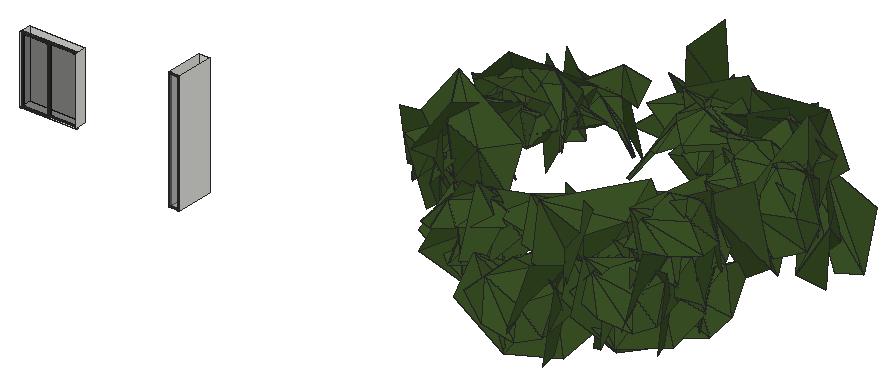
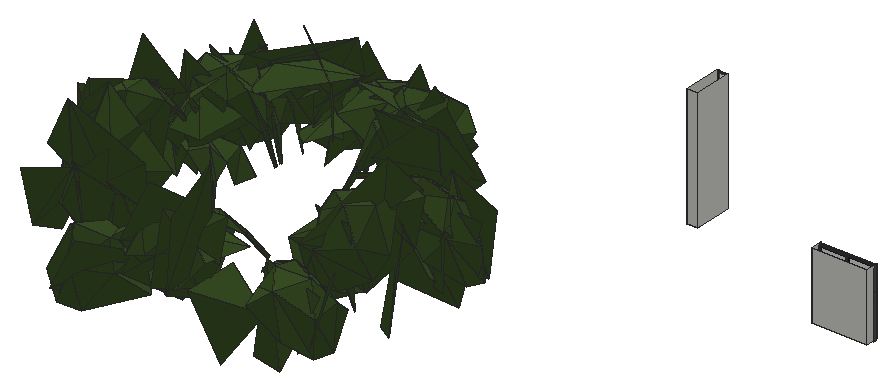
# SketchUp Ruby script. Lengths in inches.
U = 1.inch
M = Sketchup.active_model
def pt(a) = Geom::Point3d.new(a.map { |v| v * U })
def face(e, loops, mat)
  f = e.add_face(loops[0].map { |a| pt(a) })
  loops[1..].each { |l| e.add_face(l.map { |a| pt(a) }).erase! }
  f.material = f.back_material = mat if mat
  f
end
# faces: each face lists its corners as indices into pts; further lists are holes
def faces(e, pts, list, mat = nil) = list.each { |f| face(e, (f[0].is_a?(Array) ? f : [f]).map { |l| l.map { |i| pts[i] } }, mat) }
# xy, xz, yz: faces in a plane at the given z, y or x. An outline is a flat list of corners, or four numbers for a rectangle; further outlines are holes
def ring(l) = l.size == 4 ? [[l[0], l[1]], [l[2], l[1]], [l[2], l[3]], [l[0], l[3]]] : l.each_slice(2).to_a
def flat(e, list, mat, &to3) = list.each { |f| face(e, (f[0].is_a?(Array) ? f : [f]).map { |l| ring(l).map { |u, v| to3.(u, v) } }, mat) }
def xy(e, z, list, mat = nil) = flat(e, list, mat) { |x, y| [x, y, z] }
def xz(e, y, list, mat = nil) = flat(e, list, mat) { |x, z| [x, y, z] }
def yz(e, x, list, mat = nil) = flat(e, list, mat) { |y, z| [x, y, z] }
def lines(e, pts, list) = list.each { |a, b| e.add_line(pt(pts[a]), pt(pts[b])) }
# prism: a flat outline (further loops are holes) pulled along v
def prism(e, loops, v, mat = nil)
  f = face(e, loops, mat); d = Geom::Vector3d.new(v.map { |x| x * U })
  f.pushpull(f.normal.samedirection?(d) ? d.length : -d.length)
end
def box(e, o, s, mat = nil) = prism(e, [[o, [o[0] + s[0], o[1], o[2]], [o[0] + s[0], o[1] + s[1], o[2]], [o[0], o[1] + s[1], o[2]]]], [0, 0, s[2]], mat)
def at(x, y, z, deg = 0) = Geom::Transformation.translation(pt([x, y, z])) * Geom::Transformation.rotation(ORIGIN, Z_AXIS, deg.degrees)
def axes(o, x, y, z) = Geom::Transformation.new([*x, 0, *y, 0, *z, 0, *pt(o).to_a, 1])
def part(name) = M.definitions.add(name)
# library, detail: a bought-in or finely detailed component or shape, given as its bounding box
def library(name, o, s) = part(name).tap { |d| box(d.entities, o, s) }
def detail(e, o, s) = box(e.add_group.entities, o, s)
def put(e, d, t, mat = nil) = e.add_instance(d, t).tap { |i| i.material = mat if mat }
def group(e, t, mat = nil) = e.add_group.tap { |g| g.transformation = t; g.material = mat if mat }.entities
root = M.entities
M.materials.add("AM113_062_Tilia").color = [58, 81, 37]
M.materials.add("Glass_Tinted_Gray").color = [0, 0, 0]
M.materials["Glass_Tinted_Gray"].alpha = 0.125
M.materials.add("[0135_DarkGray]").color = [81, 81, 81]
M.materials.add("[Color M07]").color = [58, 58, 58]
M.materials.add("[Mirror 02]").color = [229, 229, 229]
M.materials.add("[Terrazzo Light Blue]").color = [196, 214, 227]
M.materials.add("[Translucent Glass Gray]1").color = [128, 128, 128]
M.materials["[Translucent Glass Gray]1"].alpha = 0.5
c1 = part("PENTEK_RP Fineline 50S_Sliding_DoorCase_E1")
box(c1.entities,[0,0,0],[1.51,3.66,99.27],"[0135_DarkGray]")
c2 = part("PENTEK_RP Fineline 50S_SlidingDooe_Case_E2")
box(c2.entities,[0,0,0],[96.25,3.66,1.51],"[0135_DarkGray]")
c3 = part("pentek_RP Fineline 50S_SlidingDoor_Case")
put(c3.entities,c1,at(97.76,0,0))
put(c3.entities,c2,at(1.51,0,0))
put(c3.entities,c1,at(0,0,0))
put(c3.entities,c2,at(1.51,0,97.76))
c4 = part("PENTEK_RP Fineline 50S_SlidingDoor_GlazingBead_2")
box(c4.entities,[0,0,0],[0.56,0.59,94.39],"[0135_DarkGray]")
c5 = part("PENTEK_RP Fineline 50S_SlidingDoor_Glass")
box(c5.entities,[0,0,0],[46.58,0.16,94.39],"Glass_Tinted_Gray")
c6 = part("PENTEK_RP Fineline 50S_SlidingDoor_GlazingBead")
box(c6.entities,[0,0,0],[45.47,0.59,0.56],"[0135_DarkGray]")
c7 = part("PENTEK_RP Fineline 50S_SlidingDoor_Leaf_E1")
xy(c7.entities,0,[[0,0,0.93,1.97],[0.93,1.57,1.49,1.97]],"[0135_DarkGray]")
xy(c7.entities,96.25,[[0,0,0.93,0,0.93,1.57,1.49,1.57,1.49,1.97,0,1.97]],"[0135_DarkGray]")
xz(c7.entities,0,[[0,0,0.93,96.25]],"[0135_DarkGray]")
xz(c7.entities,1.57,[[0.93,0,1.49,95.32],[0.93,95.32,1.49,96.25]],"[0135_DarkGray]")
xz(c7.entities,1.97,[[0,0,1.49,96.25]],"[0135_DarkGray]")
yz(c7.entities,0,[[0,0,1.97,96.25]],"[0135_DarkGray]")
yz(c7.entities,0.93,[[0,0,1.57,0.93],[0,0.93,1.57,95.32],[0,95.32,1.57,96.25]],"[0135_DarkGray]")
yz(c7.entities,1.49,[[1.57,0,1.97,95.32],[1.57,95.32,1.97,96.25]],"[0135_DarkGray]")
c8 = part("PENTEK_RP Fineline 50S_SlidingDoor_Leaf_E2")
xy(c8.entities,0,[[0,0,0,1.57,0.56,1.57,0.56,1.97,46.02,1.97,46.02,1.57,46.58,1.57,46.58,0]],"[0135_DarkGray]")
xy(c8.entities,0.93,[[0,0,46.58,1.57]],"[0135_DarkGray]")
xy(c8.entities,1.49,[[0.56,1.57,46.02,1.97]],"[0135_DarkGray]")
xz(c8.entities,0,[[0,0,46.58,0.93]],"[0135_DarkGray]")
xz(c8.entities,1.57,[[0,0,0.56,0.93],[46.02,0,46.58,0.93],[0.56,0.93,46.02,1.49]],"[0135_DarkGray]")
xz(c8.entities,1.97,[[0.56,0,46.02,1.49]],"[0135_DarkGray]")
yz(c8.entities,0,[[0,0,1.57,0.93]],"[0135_DarkGray]")
yz(c8.entities,0.56,[[1.57,0,1.97,0.93],[1.57,0.93,1.97,1.49]],"[0135_DarkGray]")
yz(c8.entities,46.02,[[1.57,0,1.97,0.93],[1.57,0.93,1.97,1.49]],"[0135_DarkGray]")
yz(c8.entities,46.58,[[0,0,1.57,0.93]],"[0135_DarkGray]")
c9 = part("PENTEK_RP Fineline S_SlidingDoor_Leaf1")
put(c9.entities,c4,at(0.93,0,0.93))
put(c9.entities,c4,at(46.96,0,0.93))
put(c9.entities,c5,at(1.49,1.42,0.93))
put(c9.entities,c6,at(1.49,0,0.93))
put(c9.entities,c5,at(1.49,0.59,0.93),"[Terrazzo Light Blue]")
put(c9.entities,c7,at(0,0,0))
put(c9.entities,c7,axes([48.44,0,0],[-1,0,0],[0,1,0],[0,0,1]))
put(c9.entities,c8,axes([0.93,0,96.25],[1,0,0],[0,1,0],[0,0,-1]))
put(c9.entities,c8,at(0.93,0,0))
put(c9.entities,c6,at(1.49,0,94.77))
c10 = part("PENTEK_RP Fineline 50S_SlidingDoor_Leaf2")
put(c10.entities,c5,at(1.49,1.42,0.93))
put(c10.entities,c6,at(1.49,0,94.77))
put(c10.entities,c4,at(46.96,0,0.93))
put(c10.entities,c5,at(1.49,0.59,0.93),"[Mirror 02]")
put(c10.entities,c4,at(0.93,0,0.93))
put(c10.entities,c7,at(0,0,0))
put(c10.entities,c7,axes([48.44,0,0],[-1,0,0],[0,1,0],[0,0,1]))
put(c10.entities,c6,at(1.49,0,0.93))
put(c10.entities,c8,axes([0.93,0,96.25],[1,0,0],[0,1,0],[0,0,-1]))
put(c10.entities,c8,at(0.93,0,0))
c11 = part("PENTEK - Slimmest Steel Sliding Door / Window\#1")
put(c11.entities,c3,at(0,-1.88,-0.09))
put(c11.entities,c9,at(1.51,-2.27,1.42))
put(c11.entities,c10,at(49.32,-0.3,1.42))
xy(root,364.43,[[748.74,187.1875,835.24,205.25]])
xy(root,385.18,[[1069.1,76.875,1085.03,135.5625]])
xz(root,135.5625,[[1069.1,385.18,1085.03,573.56]])
xz(root,205.25,[[748.74,364.43,835.24,469.24]])
yz(root,748.74,[[187.1875,364.43,205.25,469.24]])
yz(root,835.24,[[187.1875,364.43,205.25,469.24]])
yz(root,1069.1,[[76.875,385.18,135.5625,573.56]])
yz(root,1085.03,[[76.875,385.18,135.5625,573.56]])
p = [[1601.66,670.05,315.71],[1535.19,617.43,338.79],[1570.96,643.52,366.44],[1625.2,663.5,363.78],[1636.98,674.35,317.65],[1388.25,576.26,422.85],
  [1368.51,625.96,315.85],[1296.01,666.29,337.2],[1765.14,494.74,417.32],[1767.15,483.72,335.45],[1693.84,517.9,316.28],[1742.78,543.34,368.28],
  [1652.85,574.14,340.89],[1703.04,582.55,389.63],[1654.68,619.59,398.42],[1670.24,652.85,344.19],[1645.27,677.9,337.1],[1638.875,646.55,318.57],
  [1562.81,603.03,365.35],[1550.61,126.34,327.61],[1607.76,173.62,320.07],[1584.99,185.92,394.59],[1632.27,212.19,354.9],[1494.79,518.05,415.15],
  [1518.4,576.83,320.1],[1567.5,634.51,364.77],[1718.69,297.5,343.21],[1700.85,322.07,320.5625],[1674.8125,395.71,389.96],[1258.11,500.08,324.84],
  [1286.59,480.71,321.65],[1303.39,429.125,419.68],[1423.13,686.08,413.52],[1379.43,677.28,322.26],[1363.88,610.22,368.5],[1608.4,154.5625,428.45],
  [1603.09,137.5,323.07],[1587.13,213.46,323.94],[1516.89,225.75,399.9],[1288.65,431.48,446.63],[1247.38,501.07,412.7],[1597.91,264.72,424.69],
  [1625.4,209.625,325.1875],[1680.58,154.3,367.03],[1769.1,555.18,326.7],[1737.84,539.3,325.58],[1682.1,561.27,420.41],[1646.29,304.4,370.83],
  [1625.85,301.11,333.03],[1686.87,287.42,326.52],[1725.04,310.375,330.14],[1691.04,576.2,445.47],[1773.78,574.375,413.38],[1469.72,170.77,422.23],
  [1490.48,104.93,394.76],[1541.38,150.75,408.42],[1663.53,205.61,333.17],[1700.96,267.25,329.79],[1704.03,254,409.65],[1721.88,306.1,369.74],
  [1704.59,315.17,372.82],[1734.14,342.09,347.42],[1225.58,360.61,435.27],[1313.79,419.67,482.16],[1228.52,400.43,332.93],[1307.93,423.96,355.1875],
  [1613.39,357.38,350.35],[1626.87,187.84,462.78],[1639.87,146.86,400.84],[1681.07,200.9,418.12],[1439.32,298.77,409.11],[1425.78,220.58,333.42],
  [1388.96,163.09,397.87],[1549.89,613.46,391.29],[1608.71,674.28,414.01],[1280.33,606.87,419.91],[1234.57,326.47,437.49],[1264.04,336.34,337.34],
  [1329.94,331.53,389.87],[1564.29,582.95,348.02],[1647.49,612.625,389.11],[1719.52,233.81,451],[1722.9,212.14,346.91],[1690.75,282.64,341],
  [1616.17,281.89,411.53],[1568.19,558.3125,440.2],[1589.87,592.96,377.59],[1516.22,611.3,341.24],[1535.58,612.72,424.31],[1451.16,629.41,369.72],
  [1480.18,620.86,440.14],[1673.99,189.84,349.09],[1719.7,248.24,341.43],[1691.43,257.9375,413.42],[1733.58,292.52,374.71],[1679.28,395.6,423.1],
  [1702.47,312.47,428.94],[1264.88,389.9,343.52],[1293.98,322.24,357.18],[1279.33,340.77,432.95],[1254.625,392.125,430.01],[1281.79,455.85,467.66],
  [1233.84,453.41,398.03],[1677.46,596.53,378.62],[1287.35,392.07,344.6],[1319.96,330.07,366.98],[1273.49,331.62,422.55],[1239.48,376.71,404.25],
  [1230.04,429.5,453.05],[1223.04,438.95,371.3125],[1262.38,602.96,347.14],[1302,526.54,359.86],[1285.3,565.21,392.62],[1276.39,622.3125,395.66],
  [1265.31,638.27,351.76],[1705.51,369.11,399.71],[1705.13,417.45,387.94],[1564.97,589.41,384.97],[1581.18,218.74,435.13],[1617.01,158.18,414.03],
  [1655.99,214.55,427.25],[1264.67,646.09,372.04],[1292.9,634.69,349.57],[1323.18,549.45,386.32],[1616.08,368.72,385.01],[1391.64,476.33,452.83],
  [1335.63,478.77,350.45],[1280.36,539.07,370.66],[1585.57,435.39,350.72],[1604.83,403.7,377.875],[1604.74,409.84,382.41],[1584.52,437.68,355.09],
  [1607.68,413.98,377.85],[1587.64,437.3,351.69],[1327.25,640.92,426.85],[1294.54,665.33,377.74],[1220.4,361.4,353.94],[1241.56,335.31,369.2],
  [1222.06,364.74,404.26],[1233.16,418.33,433.74],[1214.02,404.07,368.66],[1583.85,259.21,376.45],[1482.16,316.45,355.26],[1462.08,300.06,398.92],
  [1468.16,303.3,400.95],[1484.33,319.43,357.95],[1532.14,622.18,355.55],[1529.99,584.35,426.53],[1542.81,513.3,405.51],[1586.88,566.51,383.75],
  [1479.88,607.55,439.7],[1467.48,649.55,382.49],[1472.61,300.4,396.875],[1484.76,315.51,356.46],[1306.25,288.28,407.37],[1581.24,94.3125,385.79],
  [1564.62,116.63,358.24],[1570.03,207.07,394.39],[1342.03,547.88,366.84],[1208.16,368.77,367.125],[1241.39,378.91,360.93],[1300.24,349.56,449.09],
  [1508.1,240.0625,391.63],[1488.41,261.07,361.97],[1486.29,263.08,365.69],[1485.875,259.68,362.48],[1503.34,231.51,397.07],[1505.48,238.16,398.42],
  [1577.39,323.99,456.07],[1638.76,295.3,363.48],[1708.23,269.65,416.27],[1435.09,191.16,363.8125],[1503.95,190.71,391.68],[1474.54,205.89,461.42],
  [1374.54,250.24,451.29],[1358.72,201.55,400.8],[1417.48,200.66,448.07],[1595.1,622.46,399],[1532.41,614.52,464.8],[1587.01,101.26,366.35],
  [1605.71,131.5625,365.35],[1577.94,121.21,408.27],[1595.55,176.3,407.89],[1602.49,217.8125,375.05],[1574.79,535.65,385.54],[1571.4,502.35,365.68],
  [1570.97,500.24,370.19],[1520.57,127.52,425.875],[1545.72,90.35,383.06],[1577.64,536.11,392.6],[1574.03,501.36,366.7],[1584.25,538.25,390.93],
  [1338.11,547.94,404.39],[1693.28,210.28,454.45],[1322.7,292.3,416.47],[1291.05,336.97,476.0625],[1207.625,352.55,455.01],[1663.31,408.05,367.57],
  [1656.15,396.18,400.97],[1445.13,571.04,394.78],[1245.92,446.9,411.12],[1309.53,315.45,433.6],[1263.67,333.12,436.22],[1604.86,293.59,401.65],
  [1582.46,308.61,369.28],[1579.78,310.24,372.7],[1751.94,443.61,480.73],[1642.16,438.74,509.95],[1737.29,428.61,369.4],[1656.62,451.03,385.01],
  [1465.72,517.95,409.37],[1445.1,498.82,373.08],[1447.6,500.78,369.61],[1472.08,519.52,406.34],[1697.04,311.28,432.07],[1580.27,306.72,369.73],
  [1601.84,284.41,407.4375],[1602.41,291.41,408.41],[1419.86,630.49,425.01],[1300.82,483.55,369.86],[1278.52,429.61,422.125],[1287.83,473.71,477.81],
  [1299.43,522.05,440.98],[1355.44,554.08,445.47],[1322.98,561.29,375.77],[1461.75,520.87,404.77],[1445.32,502.35,370.5625],[1296.91,528.91,480.64],
  [1668.81,352.15,406.64],[1556.9375,216.48,371.11],[1554.96,215.33,408.88],[1312.01,537.52,412.53],[1265.65,605.73,445.86],[1641.91,388.45,460.29],
  [1714.7,393.59,374.57],[1781.36,359.46,425.33],[1675.17,328.42,389.66],[1392.61,547.12,399.33],[1423.26,538.35,375.49],[1425.51,537.3,379.7],
  [1290.7,502.66,376.6],[1259.22,449.2,426.83],[1301.1,472.66,478.11],[1327.39,515.85,446.6],[1399.34,519.33,424.6875],[1349.125,558.6,384],
  [1393.16,549.64,406.58],[1424.81,540.68,376.55],[1392.28,556.61,405.57],[1353.09,659.76,405.88],[1633.42,381.25,407.04],[1629.18,562.33,379.65],
  [1504.71,632.77,478.4],[1501.32,661.26,378.85],[1441.46,613.78,380.15],[1606.875,566.03,403.67],[1634.84,267.36,499.13],[1672.66,241.71,440.52],
  [1672.82,309.09,379.7],[1680.65,307.32,467.22],[1676.19,365.33,464.52],[1676.25,381.04,385.3],[1524.27,281.84,488.5625],[1553.79,239.87,379.81],
  [1604.29,176.65,411.66],[1472.43,532.54,415.01],[1708.15,167.55,411.41],[1688.36,184.6,381.23],[1672.26,275.23,410.69],[1421.62,180.09,382.35],
  [1491.87,170.3,411.32],[1472.2,218.81,457.24],[1390.39,292.71,402.23],[1356.59,228.91,399.24],[1417.5,229.69,441.87],[1431.13,643.96,430.41],
  [1492.6,121.69,397.9],[1650.1,393.83,484.82],[1697.65,379.25,417.23],[1712.02,455.94,383.21],[1711.12,435.41,466.64],[1718.63,490.15,484.9],
  [1723.84,524.64,416.76],[1708.74,388.08,477.79],[1717.04,388.81,395.36],[1692.14,466.68,383.86],[1734.54,443.15,445.94],[1729.47,495.77,477.41],
  [1697.14,531.5,424.27],[1635.79,633.12,485.09],[1648.33,606.45,384.14],[1589.39,561.09,412.77],[1582.96,578.87,408.29],[1671.33,422.24,429.7],
  [1581.32,213.27,423.64],[1587.44,132.18,461.36],[1658.51,280.65,385.97],[1655.12,280.48,423.6],[1703.2,251.39,428.06],[1702.43,292.16,392.56],
  [1670.26,599.85,450.93],[1559.45,647.82,419.6875],[1541.1,630.73,389.0625],[1467.18,585.82,434.43],[1547.81,199.43,509.98],[1561.78,166.97,440.45],
  [1591.24,232.68,389.22],[1604.55,215.36,472.72],[1630.29,267.41,478.3],[1631.57,291.6,402.74],[1518.15,537.95,391.57],[1572.07,559.95,389.5],
  [1561.61,573.57,429.31],[1576.06,621.14,399.09],[1713.15,174.88,391.86],[1724.8125,208.49,389.67],[1698.05,193.85,431.58],[1325.45,395.8,475.43],
  [1683.36,568.96,404.87],[1614.29,594.09,389.97],[1617.875,590.85,471.39],[1570.42,607.75,424.26],[1496.06,180.52,391.01],[1508.32,198.03,416.85],
  [1531.89,209.56,426.9375],[1503.15,533.95,422.93],[1536.27,205.17,444.12],[1639.98,187.97,445.16],[1674.54,155.74,406.84],[1312.66,583.125,424.0625],
  [1763.06,475.78,493.04],[1742.72,499.44,392.96],[1685.93,532.51,446.24],[1419.57,270.93,393.28],[1370.15,239.07,401.87],[1383.92,234.73,444.23],
  [1434.25,283.1,421.96],[1670.07,551.12,399.75],[1600.49,569.6875,393.67],[1617.89,601.54,460.71],[1560.3125,592.9,429.08],[1694.55,351.99,508.45],
  [1719.61,341.7,406.39],[1658.79,389,394.26],[1586.52,348.55,447.3125],[1373.47,493.82,420.2],[1354.72,545.6,395.68],[1339.97,545.97,437.07],
  [1293.75,554.8,400.46],[1453.08,196.39,504.67],[1460.4,151.93,413.8],[1510.71,209.55,396.82],[1464.45,288.84,411.17],[1454.04,278.78,445.71],
  [1475.36,261.26,445.95],[1583.64,275.02,462.16],[1645.96,240.03,448.61],[1687.61,299.03,397.53],[1651.36,306.9375,470.84],[1662.96,362.63,465.5],
  [1700.24,372.3125,400.7],[1421.67,206.58,488.41],[1366.52,397.49,493.72],[1315.11,356.98,398.43],[1274.56,292,444.78],[1548.3,356.42,398.5],
  [1573.36,344.32,440.15],[1570.41,350.68,441.31],[1545.86,359.08,401.35],[1572.26,354.21,435.21],[1549.35,359.14,398.55],[1446.13,689.17,510.02],
  [1472.2,582.72,527.85],[1458.52,683.48,398.6],[1452.32,600.7,407.36],[1547.43,654.06,405.82],[1353.4,562.34,427.48],[1675.64,595.55,466.3125],
  [1706.27,565.39,530.3],[1737.54,565.23,457.61],[1370.41,583.49,422.88],[1376.98,605.82,399.94],[1259.12,530.93,416.82],[1387.78,295.65,400.56],
  [1431.625,284.31,438.27],[1378.4,291.29,481.23],[1319.71,319.04,407.31],[1687.39,415.4375,437.03],[1714.11,401.71,462.32],[1743.91,412.17,402.95],
  [1763.47,452.26,401.26],[1755.51,442.96,449.28],[1758.87,482.85,424.04],[1633.07,270.43,440.64],[1504.98,236.16,487],[1538.89,177.56,454.53],
  [1600.21,214.41,401.88],[1378.38,180.49,428.83],[1579.74,228.93,483.22],[1617.73,271.47,482.08],[1648.84,270.27,410.98],[1532.89,258.59,434.73],
  [1652.36,323.1,452.41],[1690,389.32,432.02],[1259.73,369.1,460.46],[1485.97,545.67,445.05],[1468.58,566.3,440.91],[1606.14,232.9,404.86],
  [1615.28,175.09,416],[1613.09,253.62,430.02],[1670.16,573.5625,490.53],[1687.44,509.47,536.05],[1733.97,547.04,483.78],[1412.97,577.96,430.95],
  [1541.62,627.64,441.3125],[1513.63,655.99,417.61],[1321.96,302.47,492.76],[1299.15,353.42,537.28],[1259.75,330.78,478.33],[1347.33,322.41,464.8125],
  [1559.12,172.86,431.13],[1459.53,576.41,407.97],[1486.76,617.36,455.88],[1441.59,612.21,434.37],[1680.5625,284.84,440.07],[1663.17,308.4,454.9],
  [1296.42,427.9375,442.48],[1527.78,190.9,454.18],[1702.49,208.59,484.25],[1615.45,218.89,511.41],[1615.68,518.9,513.36],[1467.56,210.8,476.58],
  [1511.18,220.52,450.07],[1485.81,247.36,415.41],[1682.63,318.78,505.81],[1307.81,310.18,480.15],[1727.625,551.32,475.76],[1255.03,501.8,441.45],
  [1284.66,532.64,454.05],[1463.06,585.3,467.12],[1538.625,617.82,495.13],[1376.16,486.95,456.17],[1439.5,240.12,471.28],[1274.86,413.3125,487.12],
  [1508.27,583.51,458.3],[1667.41,240.84,449.28],[1735.47,486.99,490.17],[1707.51,527.39,493.33],[1710.96,555.98,483.61],[1553.3,553.59,476],
  [1326.81,405.54,497.88],[1433.64,594.68,473.52],[1741.48,376.66,525.26],[1262.01,426,487.14],[1413.5,155.01,442.32],[1566.59,590.47,498.94],
  [1390.1,447.36,458.97],[1408.47,418.06,433.59],[1406.71,419.6875,429.2],[1388.95,452.74,453.48],[1640.27,410.86,485.6875],[1387.02,442.62,456.05],
  [1404.99,417.84,430.96],[1626.71,369.06,431.44],[1619.58,364.72,467.77],[1674.63,361.38,482.44],[1658.53,399.29,447.74],[1655.71,428.27,468.6875],
  [1320.31,359.73,437.61],[1297.71,411.4,473.625],[1603.34,344.38,479.59],[1304.63,361.86,469.52],[1617.95,418.59,439.28],[1326.52,502.86,485.51],
  [1601.94,301.25,437.99],[1636.17,253.95,450.35],[1648.13,274.83,484.66],[1595.24,320.98,464.55],[1433.57,310.83,499.74],[1294.26,435.26,488.14],
  [1291.5,483.58,490.29],[1414.6875,187.99,469.59],[1447.75,161.52,451.73],[1516.3,245.9,483.27],[1335.06,293.24,528.64],[1310.77,436.29,529.3],
  [1646.27,465.49,510.56],[1718.16,336.44,448.91],[1697.8,265.34,454.17],[1723.83,301.29,448.13],[1697.2,308.15,484.14],[1716.68,452.22,503.125],
  [1624.91,320.99,513.19],[1363.15,476.59,483.52],[1605.88,344.9,474.09],[1341.6,460.13,485.63],[1331.41,444.11,457.49],[1297.84,385.6,485.42],
  [1660.8,437.61,503.9],[1646.23,333.88,495.34],[1342.5625,400.49,479.15],[1376.25,413.95,470.87],[1376.9,415.45,475.73],[1375.48,416.76,470.875],
  [1334.4,407.34,479.16],[1338.86,403.51,484.22],[1669.5,538.38,522.08],[1707.44,523.68,540.18],[1673.89,497.27,484.31],[1682.68,481.95,514.58],
  [1593.82,477.48,500.5],[1632.17,460.6875,510.89],[1630.11,465.52,516.99],[1592.91,478.6,505.625],[1629.19,470.79,512.99],[1594.73,480.17,501.33],
  [1673.75,456.66,522.98]]
faces(root,p,[[0,1,2],[3,0,2],[4,0,3],[5,6,7],[8,9,10],[10,11,8],[10,12,13],[13,11,10],
  [4,3,14],[14,15,4],[16,17,18],[19,20,21],[20,22,21],[23,24,25],[26,27,28],[29,30,31],
  [32,33,34],[35,36,37],[35,37,38],[31,39,29],[39,40,29],[41,42,43],[44,45,46],[47,48,49],
  [47,49,50],[46,51,44],[51,52,44],[53,54,19],[19,55,53],[21,55,19],[56,57,58],[57,59,58],
  [50,60,47],[50,61,60],[62,63,64],[63,65,64],[66,48,47],[67,68,56],[56,69,67],[58,69,56],
  [70,71,72],[18,73,16],[73,74,16],[75,5,7],[76,77,78],[2,1,79],[12,80,13],[81,82,83],
  [81,83,84],[85,86,87],[87,88,85],[87,89,90],[90,88,87],[91,92,93],[92,94,93],[28,95,26],
  [95,96,26],[97,98,99],[99,100,97],[101,102,97],[97,100,101],[14,103,15],[104,105,106],[106,107,104],
  [104,107,108],[108,109,104],[110,111,112],[113,110,112],[114,110,113],[60,61,115],[61,116,115],[79,117,2],
  [118,119,91],[91,120,118],[93,120,91],[121,122,123],[47,124,66],[125,126,127],[128,129,130],[130,131,128],
  [132,133,131],[114,113,134],[134,135,114],[136,137,138],[139,140,136],[136,138,139],[21,22,141],[131,130,132],
  [142,143,144],[144,145,142],[146,147,148],[148,149,146],[150,147,146],[146,151,150],[152,153,145],[98,154,99],
  [145,144,152],[155,156,157],[112,111,158],[159,160,161],[162,163,164],[165,166,167],[167,164,165],[168,169,170],
  [171,172,173],[174,175,171],[171,176,174],[173,176,171],[14,3,177],[177,3,2],[178,23,25],[179,180,181],
  [181,180,182],[180,183,182],[164,167,162],[184,185,186],[187,188,179],[179,181,187],[177,2,117],[189,186,190],
  [190,191,189],[158,192,112],[193,41,43],[105,194,106],[195,196,159],[161,195,159],[197,198,115],[115,116,197],
  [8,11,13],[32,34,199],[139,200,140],[137,201,202],[138,137,202],[203,204,205],[206,207,208],[207,209,208],
  [210,211,212],[212,213,210],[58,59,214],[215,216,217],[217,205,215],[89,218,90],[219,220,221],[221,222,219],
  [219,222,223],[223,224,219],[186,189,184],[225,226,211],[227,125,127],[124,47,228],[47,60,228],[229,230,182],
  [182,183,229],[123,231,121],[231,232,121],[205,217,203],[228,60,115],[211,210,225],[233,234,235],[93,94,236],
  [237,238,239],[21,141,53],[240,241,242],[242,243,240],[244,245,240],[240,243,244],[246,239,247],[247,248,246],
  [134,249,135],[129,124,250],[132,130,250],[250,130,129],[250,198,132],[251,103,14],[252,253,254],[14,255,251],
  [256,257,258],[258,259,256],[260,259,258],[258,261,260],[239,246,237],[262,263,264],[252,254,265],[266,267,268],
  [269,270,271],[272,273,269],[269,274,272],[271,274,269],[151,275,150],[187,276,188],[277,278,279],[279,280,277],
  [281,280,279],[279,282,281],[283,284,285],[285,286,283],[287,286,285],[285,288,287],[289,290,291],[228,250,124],
  [292,117,184],[177,117,292],[261,293,260],[184,189,292],[157,294,155],[294,295,155],[296,297,298],[298,299,296],
  [13,80,300],[301,302,303],[304,305,306],[306,307,304],[308,307,306],[306,309,308],[310,311,312],[312,311,313],
  [13,300,8],[314,315,316],[316,315,298],[315,299,298],[93,236,118],[76,78,317],[318,319,320],[319,321,320],
  [292,189,191],[191,255,292],[322,276,187],[187,323,322],[162,167,324],[324,230,162],[312,325,310],[172,326,173],
  [327,328,314],[314,316,327],[329,112,192],[329,113,112],[330,331,332],[333,334,335],[335,336,333],[337,338,339],
  [338,340,339],[341,342,343],[341,343,344],[53,55,21],[345,346,347],[347,346,348],[134,113,329],[349,350,351],
  [349,351,352],[353,354,152],[152,144,353],[166,323,324],[324,167,166],[355,356,357],[357,358,355],[359,358,357],
  [357,360,359],[361,70,72],[362,363,364],[255,14,177],[365,366,367],[367,368,365],[369,370,368],[371,372,373],
  [372,374,373],[143,336,353],[353,144,143],[177,292,255],[312,313,375],[376,192,237],[237,246,376],[228,115,198],
  [339,377,337],[378,379,337],[337,377,378],[134,380,381],[381,249,134],[347,348,382],[383,384,385],[386,383,385],
  [360,387,359],[228,198,250],[368,367,369],[388,389,390],[390,391,388],[390,392,391],[203,217,393],[393,297,203],
  [394,395,396],[335,334,397],[396,398,394],[399,398,396],[396,400,399],[271,401,272],[272,274,271],[309,402,308],
  [388,403,389],[108,107,106],[404,138,202],[139,138,404],[329,192,376],[225,210,405],[405,406,225],[407,408,327],
  [327,409,407],[318,410,411],[411,412,318],[320,410,318],[150,413,148],[148,147,150],[376,246,248],[248,380,376],
  [375,414,312],[375,415,414],[405,210,213],[213,325,405],[327,408,328],[385,416,386],[386,416,417],[417,418,386],
  [216,409,393],[393,217,216],[99,154,419],[420,181,182],[420,182,230],[421,406,422],[422,423,421],[187,181,420],
  [420,230,324],[58,214,67],[67,69,58],[268,424,266],[400,425,399],[426,200,139],[270,427,271],[424,428,266],
  [429,262,264],[289,291,430],[118,120,93],[431,432,433],[433,354,431],[434,168,170],[106,194,435],[323,187,420],
  [420,324,323],[282,436,281],[382,437,438],[382,438,347],[415,423,422],[414,415,422],[303,439,301],[439,440,301],
  [347,441,345],[336,335,442],[442,353,336],[220,443,221],[106,435,108],[444,405,325],[325,312,444],[329,376,380],
  [380,134,329],[445,297,393],[445,298,297],[391,392,446],[392,447,446],[288,448,287],[320,321,449],[85,88,90],
  [242,450,244],[244,243,242],[90,218,451],[452,233,235],[241,453,242],[445,316,298],[335,397,454],[339,340,455],
  [456,457,458],[458,459,456],[312,414,444],[260,293,460],[409,327,445],[445,393,409],[101,100,99],[150,275,413],
  [461,462,457],[463,464,465],[465,466,463],[327,316,445],[467,403,388],[99,419,101],[202,201,468],[457,456,461],
  [469,139,404],[139,469,426],[271,427,401],[369,367,470],[470,464,369],[404,202,471],[468,471,202],[359,387,472],
  [441,347,473],[347,438,473],[474,475,476],[476,477,474],[385,384,478],[359,472,355],[90,451,85],[366,477,470],
  [470,367,366],[444,406,405],[444,422,406],[223,222,221],[444,414,422],[437,479,480],[438,437,480],[454,481,335],
  [454,482,481],[173,326,483],[335,481,442],[484,362,364],[221,485,223],[442,354,353],[442,431,354],[283,286,287],
  [330,332,486],[487,466,465],[174,176,173],[476,488,489],[489,490,476],[489,487,490],[490,487,465],[388,391,491],
  [491,391,446],[482,432,431],[476,475,488],[173,483,174],[481,482,431],[308,402,492],[493,456,459],[459,441,493],
  [473,438,480],[399,425,494],[493,495,461],[461,456,493],[473,493,441],[480,479,496],[496,495,480],[404,471,497],
  [404,497,469],[339,455,378],[378,377,339],[355,358,359],[388,498,467],[498,388,491],[260,460,256],[256,259,260],
  [477,476,499],[499,470,477],[277,280,281],[499,464,470],[499,465,464],[497,471,500],[442,481,431],[500,501,502],
  [503,504,505],[505,502,503],[320,449,411],[411,410,320],[304,307,308],[504,469,497],[399,494,394],[502,505,500],
  [281,436,506],[287,507,283],[287,448,507],[221,443,485],[242,453,450],[308,492,304],[500,505,497],[497,505,504],
  [385,478,417],[417,416,385],[394,398,399],[499,490,465],[473,495,493],[476,490,499],[508,509,446],[446,447,508],
  [281,506,277],[473,480,495],[491,446,509],[510,511,512],[512,513,510],[514,515,513],[491,516,498],[491,509,516],
  [511,498,516],[513,512,514],[516,512,511],[516,509,514],[514,512,516]],"AM113_062_Tilia")
put(root,c11,axes([748.74,190.01,362.65],[0.87134,0,0],[0,0.62,0],[0,0,1.07472]))
g1 = group(root,at(1069.1,76.875,385.18),"[Color M07]")
xy(g1,0,[[0,0,15.93,0.25]],"[Color M07]")
xy(g1,1.75,[[1.75,0,14.18,0.25]],"[Color M07]")
xy(g1,186.62,[[1.75,0,14.18,0.25]],"[Color M07]")
xy(g1,188.375,[[0,0,15.93,0.25]],"[Color M07]")
xz(g1,0,[[[0,0,15.93,188.375],[1.75,1.75,14.18,186.62]]],"[Color M07]")
xz(g1,0,[[1.75,1.75,14.18,186.62]],"[Translucent Glass Gray]1")
xz(g1,0.25,[[[0,0,15.93,188.375],[1.75,1.75,14.18,186.62]]],"[Color M07]")
yz(g1,0,[[0,0,0.25,188.375]],"[Color M07]")
yz(g1,1.75,[[0,1.75,0.25,186.62]],"[Color M07]")
yz(g1,14.18,[[0,1.75,0.25,186.62]],"[Color M07]")
yz(g1,15.93,[[0,0,0.25,188.375]],"[Color M07]")
